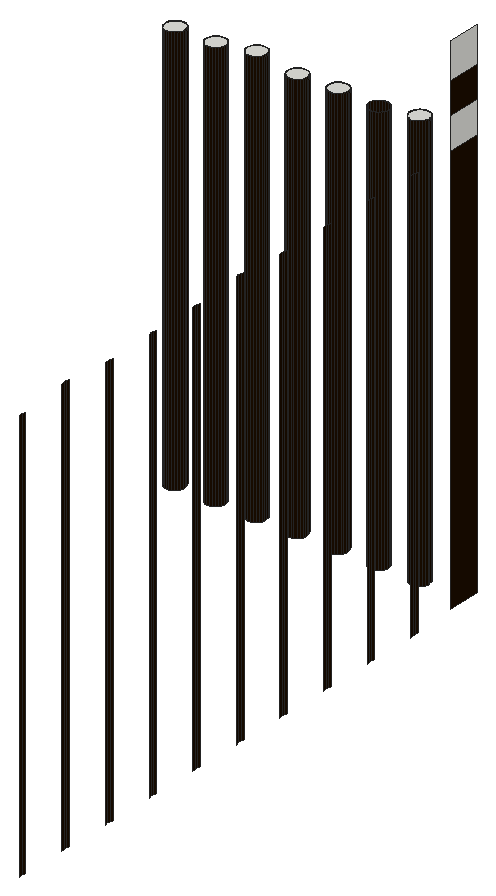
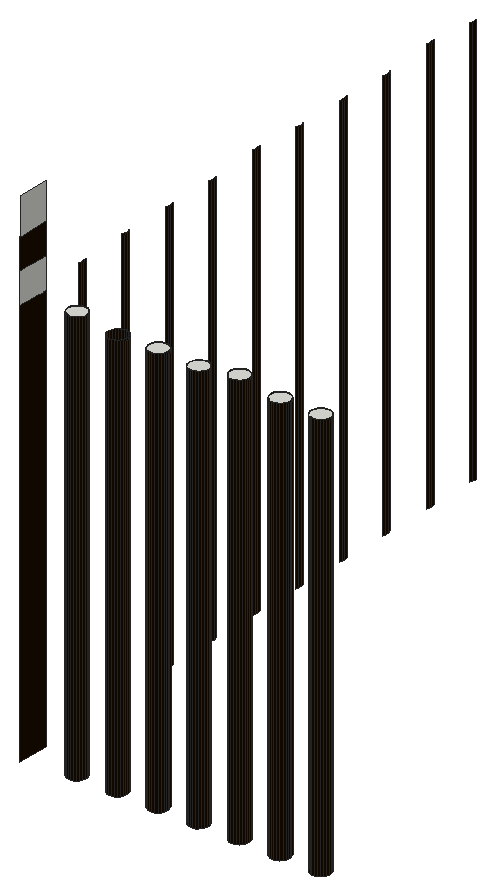
# SketchUp Ruby script. Lengths in inches.
U = 1.inch
M = Sketchup.active_model
def pt(a) = Geom::Point3d.new(a.map { |v| v * U })
def face(e, loops, mat)
  f = e.add_face(loops[0].map { |a| pt(a) })
  loops[1..].each { |l| e.add_face(l.map { |a| pt(a) }).erase! }
  f.material = f.back_material = mat if mat
  f
end
# faces: each face lists its corners as indices into pts; further lists are holes
def faces(e, pts, list, mat = nil) = list.each { |f| face(e, (f[0].is_a?(Array) ? f : [f]).map { |l| l.map { |i| pts[i] } }, mat) }
# xy, xz, yz: faces in a plane at the given z, y or x. An outline is a flat list of corners, or four numbers for a rectangle; further outlines are holes
def ring(l) = l.size == 4 ? [[l[0], l[1]], [l[2], l[1]], [l[2], l[3]], [l[0], l[3]]] : l.each_slice(2).to_a
def flat(e, list, mat, &to3) = list.each { |f| face(e, (f[0].is_a?(Array) ? f : [f]).map { |l| ring(l).map { |u, v| to3.(u, v) } }, mat) }
def xy(e, z, list, mat = nil) = flat(e, list, mat) { |x, y| [x, y, z] }
def xz(e, y, list, mat = nil) = flat(e, list, mat) { |x, z| [x, y, z] }
def yz(e, x, list, mat = nil) = flat(e, list, mat) { |y, z| [x, y, z] }
def lines(e, pts, list) = list.each { |a, b| e.add_line(pt(pts[a]), pt(pts[b])) }
# prism: a flat outline (further loops are holes) pulled along v
def prism(e, loops, v, mat = nil)
  f = face(e, loops, mat); d = Geom::Vector3d.new(v.map { |x| x * U })
  f.pushpull(f.normal.samedirection?(d) ? d.length : -d.length)
end
def box(e, o, s, mat = nil) = prism(e, [[o, [o[0] + s[0], o[1], o[2]], [o[0] + s[0], o[1] + s[1], o[2]], [o[0], o[1] + s[1], o[2]]]], [0, 0, s[2]], mat)
def at(x, y, z, deg = 0) = Geom::Transformation.translation(pt([x, y, z])) * Geom::Transformation.rotation(ORIGIN, Z_AXIS, deg.degrees)
def axes(o, x, y, z) = Geom::Transformation.new([*x, 0, *y, 0, *z, 0, *pt(o).to_a, 1])
def part(name) = M.definitions.add(name)
# library, detail: a bought-in or finely detailed component or shape, given as its bounding box
def library(name, o, s) = part(name).tap { |d| box(d.entities, o, s) }
def detail(e, o, s) = box(e.add_group.entities, o, s)
def put(e, d, t, mat = nil) = e.add_instance(d, t).tap { |i| i.material = mat if mat }
def group(e, t, mat = nil) = e.add_group.tap { |g| g.transformation = t; g.material = mat if mat }.entities
root = M.entities
M.materials.add("[Metal Seamed]1").color = [28, 14, 0]
xy(root,618.25,[[327.39,318.74,327.11,318.8125,326.85,318.95,326.64,319.15,326.48,319.4,326.4,319.6875,326.39,319.98,326.46,320.27,326.6,320.52,326.8,320.74,327.05,320.89,327.34,320.97,327.63,320.98,327.91,320.91,328.17,320.77,328.39,320.57,328.54,320.32,328.62,320.04,328.63,319.74,328.5625,319.46,328.42,319.2,328.22,318.99,327.97,318.83,327.6875,318.75],[332.21,318.74,331.92,318.8125,331.66,318.95,331.45,319.15,331.3,319.4,331.21,319.6875,331.21,319.98,331.27,320.27,331.41,320.52,331.62,320.74,331.87,320.89,332.15,320.97,332.44,320.98,332.73,320.91,332.99,320.77,333.2,320.57,333.35,320.32,333.44,320.04,333.44,319.74,333.375,319.46,333.23,319.2,333.03,318.99,332.78,318.83,332.5,318.75],[337.02,318.74,336.73,318.8125,336.48,318.95,336.26,319.15,336.11,319.4,336.03,319.6875,336.02,319.98,336.09,320.27,336.23,320.52,336.43,320.74,336.68,320.89,336.96,320.97,337.25,320.98,337.54,320.91,337.8,320.77,338.01,320.57,338.16,320.32,338.25,320.04,338.26,319.74,338.1875,319.46,338.05,319.2,337.84,318.99,337.59,318.83,337.3125,318.75],[341.83,318.74,341.55,318.8125,341.29,318.95,341.07,319.15,340.92,319.4,340.84,319.6875,340.83,319.98,340.9,320.27,341.04,320.52,341.24,320.74,341.49,320.89,341.77,320.97,342.07,320.98,342.35,320.91,342.61,320.77,342.82,320.57,342.98,320.32,343.06,320.04,343.07,319.74,343,319.46,342.86,319.2,342.66,318.99,342.41,318.83,342.125,318.75],[346.64,318.74,346.36,318.8125,346.1,318.95,345.89,319.15,345.73,319.4,345.65,319.6875,345.64,319.98,345.71,320.27,345.85,320.52,346.05,320.74,346.3,320.89,346.59,320.97,346.88,320.98,347.16,320.91,347.42,320.77,347.64,320.57,347.79,320.32,347.87,320.04,347.88,319.74,347.8125,319.46,347.67,319.2,347.47,318.99,347.22,318.83,346.9375,318.75],
  [351.46,318.74,351.17,318.8125,350.91,318.95,350.7,319.15,350.55,319.4,350.46,319.6875,350.46,319.98,350.52,320.27,350.66,320.52,350.87,320.74,351.12,320.89,351.4,320.97,351.69,320.98,351.98,320.91,352.24,320.77,352.45,320.57,352.6,320.32,352.69,320.04,352.69,319.74,352.625,319.46,352.48,319.2,352.28,318.99,352.03,318.83,351.75,318.75],[356.27,318.74,355.98,318.8125,355.73,318.95,355.51,319.15,355.36,319.4,355.28,319.6875,355.27,319.98,355.34,320.27,355.48,320.52,355.68,320.74,355.93,320.89,356.21,320.97,356.5,320.98,356.79,320.91,357.05,320.77,357.26,320.57,357.41,320.32,357.5,320.04,357.51,319.74,357.4375,319.46,357.3,319.2,357.09,318.99,356.84,318.83,356.5625,318.75]])
xy(root,666.6875,[[327.39,318.74,327.6875,318.75,327.97,318.83,328.22,318.99,328.42,319.2,328.5625,319.46,328.63,319.74,328.62,320.04,328.54,320.32,328.39,320.57,328.17,320.77,327.91,320.91,327.63,320.98,327.34,320.97,327.05,320.89,326.8,320.74,326.6,320.52,326.46,320.27,326.39,319.98,326.4,319.6875,326.48,319.4,326.64,319.15,326.85,318.95,327.11,318.8125]])
xy(root,666.75,[[332.21,318.74,332.5,318.75,332.78,318.83,333.03,318.99,333.23,319.2,333.375,319.46,333.44,319.74,333.44,320.04,333.35,320.32,333.2,320.57,332.99,320.77,332.73,320.91,332.44,320.98,332.15,320.97,331.87,320.89,331.62,320.74,331.41,320.52,331.27,320.27,331.21,319.98,331.21,319.6875,331.3,319.4,331.45,319.15,331.66,318.95,331.92,318.8125],[341.83,318.74,342.125,318.75,342.41,318.83,342.66,318.99,342.86,319.2,343,319.46,343.07,319.74,343.06,320.04,342.98,320.32,342.82,320.57,342.61,320.77,342.35,320.91,342.07,320.98,341.77,320.97,341.49,320.89,341.24,320.74,341.04,320.52,340.9,320.27,340.83,319.98,340.84,319.6875,340.92,319.4,341.07,319.15,341.29,318.95,341.55,318.8125]])
xy(root,666.9375,[[346.64,318.74,346.9375,318.75,347.22,318.83,347.47,318.99,347.67,319.2,347.8125,319.46,347.88,319.74,347.87,320.04,347.79,320.32,347.64,320.57,347.42,320.77,347.16,320.91,346.88,320.98,346.59,320.97,346.3,320.89,346.05,320.74,345.85,320.52,345.71,320.27,345.64,319.98,345.65,319.6875,345.73,319.4,345.89,319.15,346.1,318.95,346.36,318.8125]])
xy(root,667.4375,[[356.27,318.74,356.5625,318.75,356.84,318.83,357.09,318.99,357.3,319.2,357.4375,319.46,357.51,319.74,357.5,320.04,357.41,320.32,357.26,320.57,357.05,320.77,356.79,320.91,356.5,320.98,356.21,320.97,355.93,320.89,355.68,320.74,355.48,320.52,355.34,320.27,355.27,319.98,355.28,319.6875,355.36,319.4,355.51,319.15,355.73,318.95,355.98,318.8125]])
xy(root,667.5,[[337.02,318.74,337.3125,318.75,337.59,318.83,337.84,318.99,338.05,319.2,338.1875,319.46,338.26,319.74,338.25,320.04,338.16,320.32,338.01,320.57,337.8,320.77,337.54,320.91,337.25,320.98,336.96,320.97,336.68,320.89,336.43,320.74,336.23,320.52,336.09,320.27,336.02,319.98,336.03,319.6875,336.11,319.4,336.26,319.15,336.48,318.95,336.73,318.8125]])
yz(root,331.21,[[319.6875,618.25,319.98,666.75]],"[Metal Seamed]1")
yz(root,333.44,[[319.74,618.25,320.04,666.75]],"[Metal Seamed]1")
yz(root,350.46,[[319.6875,618.25,319.98,666.66]],"[Metal Seamed]1")
yz(root,352.69,[[319.74,618.25,320.04,666.66]],"[Metal Seamed]1")
yz(root,361.97,[[317.52,674.05,321.28,678.3125]])
yz(root,361.98,[[317.52,666.66,321.28,670.37]])
yz(root,361.98,[[317.52,618.25,321.28,666.66],[317.52,670.37,321.28,674.05]],"[Metal Seamed]1")
yz(root,362.41,[[253.35,618.25,253.69,667],[259.79,618.25,260.13,667.625],[266.22,618.25,266.57,667.0625],[272.66,618.25,273,667.25],[279.1,618.25,279.44,667.25],
  [285.54,618.25,285.88,667.6875],[291.97,618.25,292.32,667.1875],[298.41,618.25,298.75,667.25],[304.85,618.25,305.19,667.1875],[311.29,618.25,311.63,667]],"[Metal Seamed]1")
p = [[362.5,254.02,618.25],[362.41,253.69,618.25],[362.41,253.69,667],[362.5,254.02,667],[362.41,259.79,618.25],[362.5,259.46,618.25],
  [362.5,259.46,667.625],[362.41,259.79,667.625],[362.5,260.46,618.25],[362.41,260.13,618.25],[362.41,260.13,667.625],[362.5,260.46,667.625],
  [362.41,266.22,618.25],[362.5,265.89,618.25],[362.5,265.89,667.0625],[362.41,266.22,667.0625],[362.5,266.9,618.25],[362.41,266.57,618.25],
  [362.41,266.57,667.0625],[362.5,266.9,667.0625],[362.41,272.66,618.25],[362.5,272.33,618.25],[362.5,272.33,667.25],[362.41,272.66,667.25],
  [362.5,273.33,618.25],[362.41,273,618.25],[362.41,273,667.25],[362.5,273.33,667.25],[362.41,279.1,618.25],[362.5,278.77,618.25],
  [362.5,278.77,667.25],[362.41,279.1,667.25],[362.5,279.77,618.25],[362.41,279.44,618.25],[362.41,279.44,667.25],[362.5,279.77,667.25],
  [362.41,285.54,618.25],[362.5,285.21,618.25],[362.5,285.21,667.6875],[362.41,285.54,667.6875],[362.5,286.21,618.25],[362.41,285.88,618.25],
  [362.41,285.88,667.6875],[362.5,286.21,667.6875],[362.41,291.97,618.25],[362.5,291.64,618.25],[362.5,291.64,667.1875],[362.41,291.97,667.1875],
  [362.5,292.65,618.25],[362.41,292.32,618.25],[362.41,292.32,667.1875],[362.5,292.65,667.1875],[362.41,298.41,618.25],[362.5,298.08,618.25],
  [362.5,298.08,667.25],[362.41,298.41,667.25],[362.5,299.08,618.25],[362.41,298.75,618.25],[362.41,298.75,667.25],[362.5,299.08,667.25],
  [362.41,304.85,618.25],[362.5,304.52,618.25],[362.5,304.52,667.1875],[362.41,304.85,667.1875],[362.5,305.52,618.25],[362.41,305.19,618.25],
  [362.41,305.19,667.1875],[362.5,305.52,667.1875],[362.41,311.29,618.25],[362.5,310.96,618.25],[362.5,310.96,667],[362.41,311.29,667],
  [362.5,311.96,618.25],[362.41,311.63,618.25],[362.41,311.63,667],[362.5,311.96,667],[327.11,318.8125,618.25],[327.39,318.74,618.25],
  [327.39,318.74,666.6875],[327.11,318.8125,666.6875],[327.6875,318.75,618.25],[327.6875,318.75,666.6875],[331.92,318.8125,618.25],[332.21,318.74,618.25],
  [332.21,318.74,666.75],[331.92,318.8125,666.75],[332.5,318.75,618.25],[332.5,318.75,666.75],[336.73,318.8125,618.25],[337.02,318.74,618.25],
  [337.02,318.74,667.5],[336.73,318.8125,667.5],[337.3125,318.75,618.25],[337.3125,318.75,667.5],[341.55,318.8125,618.25],[341.83,318.74,618.25],
  [341.83,318.74,666.75],[341.55,318.8125,666.75],[342.125,318.75,618.25],[342.125,318.75,666.75],[346.36,318.8125,618.25],[346.64,318.74,618.25],
  [346.64,318.74,666.9375],[346.36,318.8125,666.9375],[346.9375,318.75,618.25],[346.9375,318.75,666.9375],[351.17,318.8125,618.25],[351.46,318.74,618.25],
  [351.46,318.74,666.66],[351.17,318.8125,666.66],[351.75,318.75,618.25],[351.75,318.75,666.66],[355.98,318.8125,618.25],[356.27,318.74,618.25],
  [356.27,318.74,667.4375],[355.98,318.8125,667.4375],[356.5625,318.75,618.25],[356.5625,318.75,667.4375],[326.85,318.95,618.25],[326.85,318.95,666.6875],
  [327.97,318.83,618.25],[327.97,318.83,666.6875],[328.22,318.99,618.25],[328.22,318.99,666.6875],[331.66,318.95,618.25],[331.66,318.95,666.75],
  [332.78,318.83,618.25],[332.78,318.83,666.75],[333.03,318.99,618.25],[333.03,318.99,666.75],[336.48,318.95,618.25],[336.48,318.95,667.5],
  [337.59,318.83,618.25],[337.59,318.83,667.5],[337.84,318.99,618.25],[337.84,318.99,667.5],[341.29,318.95,618.25],[341.29,318.95,666.75],
  [342.41,318.83,618.25],[342.41,318.83,666.75],[342.66,318.99,618.25],[342.66,318.99,666.75],[346.1,318.95,618.25],[346.1,318.95,666.9375],
  [347.22,318.83,618.25],[347.22,318.83,666.9375],[347.47,318.99,618.25],[347.47,318.99,666.9375],[350.91,318.95,618.25],[350.91,318.95,666.66],
  [352.03,318.83,618.25],[352.03,318.83,666.66],[352.28,318.99,618.25],[352.28,318.99,666.66],[355.73,318.95,618.25],[355.73,318.95,667.4375],
  [356.84,318.83,618.25],[356.84,318.83,667.4375],[357.09,318.99,618.25],[357.09,318.99,667.4375],[326.64,319.15,618.25],[326.64,319.15,666.6875],
  [328.42,319.2,618.25],[328.42,319.2,666.6875],[331.45,319.15,618.25],[331.45,319.15,666.75],[333.23,319.2,618.25],[333.23,319.2,666.75],
  [336.26,319.15,618.25],[336.26,319.15,667.5],[338.05,319.2,618.25],[338.05,319.2,667.5],[341.07,319.15,618.25],[341.07,319.15,666.75],
  [342.86,319.2,618.25],[342.86,319.2,666.75],[345.89,319.15,618.25],[345.89,319.15,666.9375],[347.67,319.2,618.25],[347.67,319.2,666.9375],
  [350.7,319.15,618.25],[350.7,319.15,666.66],[352.48,319.2,618.25],[352.48,319.2,666.66],[355.51,319.15,618.25],[355.51,319.15,667.4375],
  [357.3,319.2,618.25],[357.3,319.2,667.4375],[326.48,319.4,618.25],[326.48,319.4,666.6875],[328.5625,319.46,618.25],[328.5625,319.46,666.6875],
  [331.3,319.4,618.25],[331.3,319.4,666.75],[333.375,319.46,618.25],[333.375,319.46,666.75],[336.11,319.4,618.25],[336.11,319.4,667.5],
  [338.1875,319.46,618.25],[338.1875,319.46,667.5],[340.92,319.4,618.25],[340.92,319.4,666.75],[343,319.46,618.25],[343,319.46,666.75],
  [345.73,319.4,618.25],[345.73,319.4,666.9375],[347.8125,319.46,618.25],[347.8125,319.46,666.9375],[350.55,319.4,618.25],[350.55,319.4,666.66],
  [352.625,319.46,618.25],[352.625,319.46,666.66],[355.36,319.4,618.25],[355.36,319.4,667.4375],[357.4375,319.46,618.25],[357.4375,319.46,667.4375],
  [326.4,319.6875,618.25],[326.4,319.6875,666.6875],[331.21,319.6875,618.25],[331.21,319.6875,666.75],[336.03,319.6875,618.25],[336.03,319.6875,667.5],
  [340.84,319.6875,618.25],[340.84,319.6875,666.75],[345.65,319.6875,618.25],[345.65,319.6875,666.9375],[350.46,319.6875,618.25],[350.46,319.6875,666.66],
  [355.28,319.6875,618.25],[355.28,319.6875,667.4375],[328.63,319.74,618.25],[328.63,319.74,666.6875],[333.44,319.74,618.25],[333.44,319.74,666.75],
  [338.26,319.74,618.25],[338.26,319.74,667.5],[343.07,319.74,618.25],[343.07,319.74,666.75],[347.88,319.74,618.25],[347.88,319.74,666.9375],
  [352.69,319.74,618.25],[352.69,319.74,666.66],[357.51,319.74,618.25],[357.51,319.74,667.4375],[326.39,319.98,618.25],[326.39,319.98,666.6875],
  [328.62,320.04,618.25],[328.62,320.04,666.6875],[336.02,319.98,618.25],[336.02,319.98,667.5],[338.25,320.04,618.25],[338.25,320.04,667.5],
  [340.83,319.98,618.25],[340.83,319.98,666.75],[343.06,320.04,618.25],[343.06,320.04,666.75],[345.64,319.98,618.25],[345.64,319.98,666.9375],
  [347.87,320.04,618.25],[347.87,320.04,666.9375],[355.27,319.98,618.25],[355.27,319.98,667.4375],[357.5,320.04,618.25],[357.5,320.04,667.4375],
  [326.46,320.27,618.25],[326.46,320.27,666.6875],[328.54,320.32,618.25],[328.54,320.32,666.6875],[331.27,320.27,618.25],[331.21,319.98,618.25],
  [331.21,319.98,666.75],[331.27,320.27,666.75],[333.44,320.04,618.25],[333.35,320.32,618.25],[333.35,320.32,666.75],[333.44,320.04,666.75],
  [336.09,320.27,618.25],[336.09,320.27,667.5],[338.16,320.32,618.25],[338.16,320.32,667.5],[340.9,320.27,618.25],[340.9,320.27,666.75],
  [342.98,320.32,618.25],[342.98,320.32,666.75],[345.71,320.27,618.25],[345.71,320.27,666.9375],[347.79,320.32,618.25],[347.79,320.32,666.9375],
  [350.52,320.27,618.25],[350.46,319.98,618.25],[350.46,319.98,666.66],[350.52,320.27,666.66],[352.69,320.04,618.25],[352.6,320.32,618.25],
  [352.6,320.32,666.66],[352.69,320.04,666.66],[355.34,320.27,618.25],[355.34,320.27,667.4375],[357.41,320.32,618.25],[357.41,320.32,667.4375],
  [326.6,320.52,618.25],[326.6,320.52,666.6875],[328.39,320.57,618.25],[328.39,320.57,666.6875],[331.41,320.52,618.25],[331.41,320.52,666.75],
  [333.2,320.57,618.25],[333.2,320.57,666.75],[336.23,320.52,618.25],[336.23,320.52,667.5],[338.01,320.57,618.25],[338.01,320.57,667.5],
  [341.04,320.52,618.25],[341.04,320.52,666.75],[342.82,320.57,618.25],[342.82,320.57,666.75],[345.85,320.52,618.25],[345.85,320.52,666.9375],
  [347.64,320.57,618.25],[347.64,320.57,666.9375],[350.66,320.52,618.25],[350.66,320.52,666.66],[352.45,320.57,618.25],[352.45,320.57,666.66],
  [355.48,320.52,618.25],[355.48,320.52,667.4375],[357.26,320.57,618.25],[357.26,320.57,667.4375],[326.8,320.74,618.25],[326.8,320.74,666.6875],
  [331.62,320.74,618.25],[331.62,320.74,666.75],[336.43,320.74,618.25],[336.43,320.74,667.5],[341.24,320.74,618.25],[341.24,320.74,666.75],
  [346.05,320.74,618.25],[346.05,320.74,666.9375],[350.87,320.74,618.25],[350.87,320.74,666.66],[355.68,320.74,618.25],[355.68,320.74,667.4375],
  [328.17,320.77,618.25],[328.17,320.77,666.6875],[332.99,320.77,618.25],[332.99,320.77,666.75],[337.8,320.77,618.25],[337.8,320.77,667.5],
  [342.61,320.77,618.25],[342.61,320.77,666.75],[347.42,320.77,618.25],[347.42,320.77,666.9375],[352.24,320.77,618.25],[352.24,320.77,666.66],
  [357.05,320.77,618.25],[357.05,320.77,667.4375],[327.05,320.89,618.25],[327.05,320.89,666.6875],[331.87,320.89,618.25],[331.87,320.89,666.75],
  [336.68,320.89,618.25],[336.68,320.89,667.5],[341.49,320.89,618.25],[341.49,320.89,666.75],[346.3,320.89,618.25],[346.3,320.89,666.9375],
  [351.12,320.89,618.25],[351.12,320.89,666.66],[355.93,320.89,618.25],[355.93,320.89,667.4375],[327.91,320.91,618.25],[327.91,320.91,666.6875],
  [332.73,320.91,618.25],[332.73,320.91,666.75],[337.54,320.91,618.25],[337.54,320.91,667.5],[342.35,320.91,618.25],[342.35,320.91,666.75],
  [347.16,320.91,618.25],[347.16,320.91,666.9375],[351.98,320.91,618.25],[351.98,320.91,666.66],[356.79,320.91,618.25],[356.79,320.91,667.4375],
  [327.34,320.97,618.25],[327.34,320.97,666.6875],[327.63,320.98,618.25],[327.63,320.98,666.6875],[332.15,320.97,618.25],[332.15,320.97,666.75],
  [332.44,320.98,618.25],[332.44,320.98,666.75],[336.96,320.97,618.25],[336.96,320.97,667.5],[337.25,320.98,618.25],[337.25,320.98,667.5],
  [341.77,320.97,618.25],[341.77,320.97,666.75],[342.07,320.98,618.25],[342.07,320.98,666.75],[346.59,320.97,618.25],[346.59,320.97,666.9375],
  [346.88,320.98,618.25],[346.88,320.98,666.9375],[351.4,320.97,618.25],[351.4,320.97,666.66],[351.69,320.98,618.25],[351.69,320.98,666.66],
  [356.21,320.97,618.25],[356.21,320.97,667.4375],[356.5,320.98,618.25],[356.5,320.98,667.4375]]
faces(root,p,[[0,1,2,3],[4,5,6,7],[8,9,10,11],[12,13,14,15],[16,17,18,19],[20,21,22,23],[24,25,26,27],[28,29,30,31],
  [32,33,34,35],[36,37,38,39],[40,41,42,43],[44,45,46,47],[48,49,50,51],[52,53,54,55],[56,57,58,59],[60,61,62,63],
  [64,65,66,67],[68,69,70,71],[72,73,74,75],[76,77,78,79],[77,80,81,78],[82,83,84,85],[83,86,87,84],[88,89,90,91],
  [89,92,93,90],[94,95,96,97],[95,98,99,96],[100,101,102,103],[101,104,105,102],[106,107,108,109],[107,110,111,108],[112,113,114,115],
  [113,116,117,114],[118,76,79,119],[80,120,121,81],[120,122,123,121],[124,82,85,125],[86,126,127,87],[126,128,129,127],[130,88,91,131],
  [92,132,133,93],[132,134,135,133],[136,94,97,137],[98,138,139,99],[138,140,141,139],[142,100,103,143],[104,144,145,105],[144,146,147,145],
  [148,106,109,149],[110,150,151,111],[150,152,153,151],[154,112,115,155],[116,156,157,117],[156,158,159,157],[160,118,119,161],[122,162,163,123],
  [164,124,125,165],[128,166,167,129],[168,130,131,169],[134,170,171,135],[172,136,137,173],[140,174,175,141],[176,142,143,177],[146,178,179,147],
  [180,148,149,181],[152,182,183,153],[184,154,155,185],[158,186,187,159],[188,160,161,189],[162,190,191,163],[192,164,165,193],[166,194,195,167],
  [196,168,169,197],[170,198,199,171],[200,172,173,201],[174,202,203,175],[204,176,177,205],[178,206,207,179],[208,180,181,209],[182,210,211,183],
  [212,184,185,213],[186,214,215,187],[216,188,189,217],[218,192,193,219],[220,196,197,221],[222,200,201,223],[224,204,205,225],[226,208,209,227],
  [228,212,213,229],[190,230,231,191],[194,232,233,195],[198,234,235,199],[202,236,237,203],[206,238,239,207],[210,240,241,211],[214,242,243,215],
  [244,216,217,245],[230,246,247,231],[248,220,221,249],[234,250,251,235],[252,222,223,253],[236,254,255,237],[256,224,225,257],[238,258,259,239],
  [260,228,229,261],[242,262,263,243],[264,244,245,265],[246,266,267,247],[268,269,270,271],[272,273,274,275],[276,248,249,277],[250,278,279,251],
  [280,252,253,281],[254,282,283,255],[284,256,257,285],[258,286,287,259],[288,289,290,291],[292,293,294,295],[296,260,261,297],[262,298,299,263],
  [300,264,265,301],[266,302,303,267],[304,268,271,305],[273,306,307,274],[308,276,277,309],[278,310,311,279],[312,280,281,313],[282,314,315,283],
  [316,284,285,317],[286,318,319,287],[320,288,291,321],[293,322,323,294],[324,296,297,325],[298,326,327,299],[328,300,301,329],[330,304,305,331],
  [332,308,309,333],[334,312,313,335],[336,316,317,337],[338,320,321,339],[340,324,325,341],[302,342,343,303],[306,344,345,307],[310,346,347,311],
  [314,348,349,315],[318,350,351,319],[322,352,353,323],[326,354,355,327],[356,328,329,357],[358,330,331,359],[360,332,333,361],[362,334,335,363],
  [364,336,337,365],[366,338,339,367],[368,340,341,369],[342,370,371,343],[344,372,373,345],[346,374,375,347],[348,376,377,349],[350,378,379,351],
  [352,380,381,353],[354,382,383,355],[384,356,357,385],[370,386,387,371],[388,358,359,389],[372,390,391,373],[392,360,361,393],[374,394,395,375],
  [396,362,363,397],[376,398,399,377],[400,364,365,401],[378,402,403,379],[404,366,367,405],[380,406,407,381],[408,368,369,409],[382,410,411,383],
  [386,384,385,387],[390,388,389,391],[394,392,393,395],[398,396,397,399],[402,400,401,403],[406,404,405,407],[410,408,409,411]],"[Metal Seamed]1")
